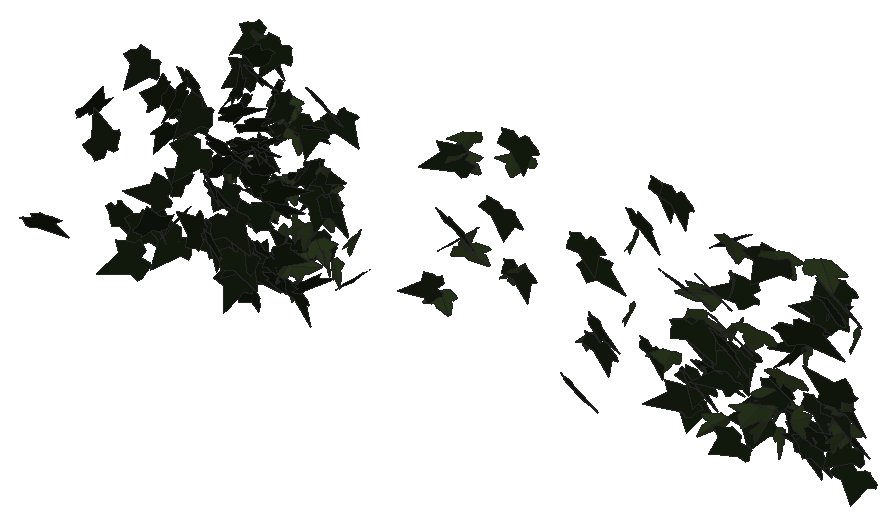
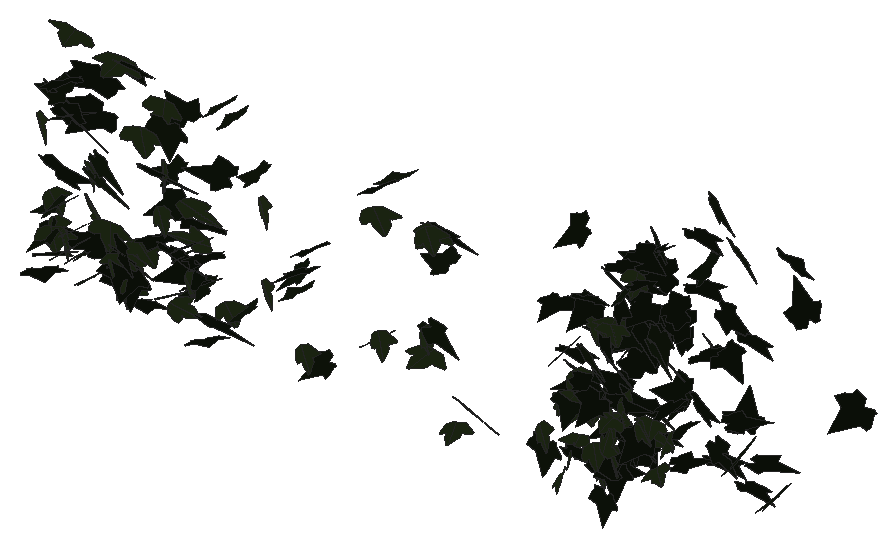
# SketchUp Ruby script. Lengths in millimetres.
U = 1.mm
M = Sketchup.active_model
def pt(a) = Geom::Point3d.new(a.map { |v| v * U })
def face(e, loops, mat)
  f = e.add_face(loops[0].map { |a| pt(a) })
  loops[1..].each { |l| e.add_face(l.map { |a| pt(a) }).erase! }
  f.material = f.back_material = mat if mat
  f
end
# faces: each face lists its corners as indices into pts; further lists are holes
def faces(e, pts, list, mat = nil) = list.each { |f| face(e, (f[0].is_a?(Array) ? f : [f]).map { |l| l.map { |i| pts[i] } }, mat) }
# xy, xz, yz: faces in a plane at the given z, y or x. An outline is a flat list of corners, or four numbers for a rectangle; further outlines are holes
def ring(l) = l.size == 4 ? [[l[0], l[1]], [l[2], l[1]], [l[2], l[3]], [l[0], l[3]]] : l.each_slice(2).to_a
def flat(e, list, mat, &to3) = list.each { |f| face(e, (f[0].is_a?(Array) ? f : [f]).map { |l| ring(l).map { |u, v| to3.(u, v) } }, mat) }
def xy(e, z, list, mat = nil) = flat(e, list, mat) { |x, y| [x, y, z] }
def xz(e, y, list, mat = nil) = flat(e, list, mat) { |x, z| [x, y, z] }
def yz(e, x, list, mat = nil) = flat(e, list, mat) { |y, z| [x, y, z] }
def lines(e, pts, list) = list.each { |a, b| e.add_line(pt(pts[a]), pt(pts[b])) }
# prism: a flat outline (further loops are holes) pulled along v
def prism(e, loops, v, mat = nil)
  f = face(e, loops, mat); d = Geom::Vector3d.new(v.map { |x| x * U })
  f.pushpull(f.normal.samedirection?(d) ? d.length : -d.length)
end
def box(e, o, s, mat = nil) = prism(e, [[o, [o[0] + s[0], o[1], o[2]], [o[0] + s[0], o[1] + s[1], o[2]], [o[0], o[1] + s[1], o[2]]]], [0, 0, s[2]], mat)
def at(x, y, z, deg = 0) = Geom::Transformation.translation(pt([x, y, z])) * Geom::Transformation.rotation(ORIGIN, Z_AXIS, deg.degrees)
def axes(o, x, y, z) = Geom::Transformation.new([*x, 0, *y, 0, *z, 0, *pt(o).to_a, 1])
def part(name) = M.definitions.add(name)
# library, detail: a bought-in or finely detailed component or shape, given as its bounding box
def library(name, o, s) = part(name).tap { |d| box(d.entities, o, s) }
def detail(e, o, s) = box(e.add_group.entities, o, s)
def put(e, d, t, mat = nil) = e.add_instance(d, t).tap { |i| i.material = mat if mat }
def group(e, t, mat = nil) = e.add_group.tap { |g| g.transformation = t; g.material = mat if mat }.entities
root = M.entities
M.materials.add("efeu1").color = [18, 25, 13]
M.materials.add("efeu2").color = [43, 57, 29]
c1 = part("ivyleaf_9")
p = [[39.1,54.8,31.7],[34.5,51.8,30.2],[-5.3,25.2,17.3],[-17.9,28.3,20.9],[-21.6,21.7,17],[-20.2,4.3,5.3],
  [-22.9,-0.3,2.5],[-17.1,-4,-0.6],[-2,-2.1,-1.2],[-0.7,-15.4,-10.1],[16.6,-22.3,-16.7],[21.1,-15.1,-12.5],
  [32.7,-10.7,-11],[46.1,-1.8,-6.6],[30.8,11.2,3.8]]
faces(c1.entities,p,[[0,1,2,3,4,5,6,7,8,9,10,11,12,13,14]],"efeu1")
c2 = part("ivyleaf_10")
p = [[0,12.8,-0.8],[-1.5,51.3,-10.9],[-4.9,51,-11.6],[-13.6,26.5,-7.3],[-13.2,15.9,-4.6],[-21.1,19.3,-7.2],
  [-29.5,16.3,-8.3],[-29.2,8.3,-6.2],[-19.7,-9.8,0.5],[-7.6,-13,4],[1,-12.2,5.8],[-0.4,51.1,-11.1],
  [-1.5,51.1,-10.9],[1,-12.4,5.9],[16.9,-12.4,3.5],[35.1,9.1,-5.1],[35,12.9,-6.1],[20.5,16.4,-4.9],
  [15.8,15,-3.8],[15.3,27.6,-7.1],[12.8,31.3,-7.8]]
faces(c2.entities,p,[[0,1,2,3,4,5,6,7,8,9,10],[11,12,0,13,14,15,16,17,18,19,20]],"efeu2")
put(root,c1,axes([93,223.6,3671.9],[1.66259,0.54862,0.30222],[0.33941,0.11819,-1.46906],[-0.68464,1.39088,0.00562]))
put(root,c1,axes([103.5,568.1,3553],[0.86385,-1.23112,-0.31612],[-0.01557,0.35496,-1.41095],[1.55061,0.68942,0.16195]))
put(root,c1,axes([180.4,600.8,4020.9],[-1.61986,-0.38705,-0.13705],[0.16378,0.02916,-1.38299],[0.4734,-1.33449,0.00953]))
put(root,c1,axes([177.8,350.7,3974.7],[0.97629,1.1061,0.65598],[-0.46966,-0.53115,1.36522],[1.49696,-0.88802,0.00051]))
put(root,c1,axes([212.5,563.8,3543.1],[-1.56561,-0.42191,0.02426],[-0.02745,-0.00923,-1.35086],[0.51485,-1.28348,0.00174]))
put(root,c1,axes([286.2,430.4,3527.5],[-1.41742,-0.52267,0.7875],[-0.87591,-0.32355,-1.27397],[0.74995,-1.36576,0.00044]))
put(root,c1,axes([299.2,523.3,3683.5],[-0.82666,-0.1305,1.15622],[-1.35744,-0.31875,-0.68804],[0.41528,-1.30168,0.05257]))
put(root,c1,axes([269.4,558.1,3580.9],[0.72765,-1.16339,-0.67837],[0.37417,-0.60509,1.30737],[-1.59984,-0.67066,-0.00278]))
put(root,c1,axes([342,503.3,4001.5],[-0.41991,0.20999,-1.38623],[-1.63505,-0.46852,0.26179],[-0.50239,1.34929,0.30664]))
put(root,c1,axes([321,522.1,3900.5],[-0.02006,1.00641,-0.92606],[0.06724,-0.92488,-1.00611],[-1.66716,-0.04941,-0.02943]))
put(root,c1,axes([330,548.8,3617.5],[-0.7977,0.991,-0.59397],[0.30979,-0.54255,-1.18473],[-1.37509,-0.69712,0.07767]))
put(root,c1,axes([341.5,530.6,3565.5],[-1.64628,-0.66672,0.05597],[-0.06226,-0.02307,-1.50513],[0.81388,-1.35037,-0.00192]))
put(root,c1,axes([324.7,436.7,3628.8],[1.05978,0.58087,1.00057],[-0.9984,-0.57596,1.04485],[0.99775,-1.19332,-0.01725]))
put(root,c1,axes([367.3,187,4002],[-1.75311,0.25356,-0.39672],[-0.49078,0.00084,1.45765],[0.29846,1.49073,0.06665]))
put(root,c1,axes([344.5,596.9,3909.2],[-0.8173,-1.09414,0.35514],[-0.1806,-0.32555,-1.28224],[1.39173,-0.68478,0.04216]))
put(root,c2,axes([359.2,722.5,3691],[-0.07252,0.88199,-0.84663],[-0.03391,-0.84839,-0.88187],[-1.49116,-0.02361,0.06123]))
put(root,c1,axes([413.5,358.1,4101.2],[-0.92706,1.06786,0.64427],[-0.41717,0.54714,-1.31017],[-1.46323,-0.83256,-0.03466]))
put(root,c1,axes([418.2,603.6,3551.2],[-0.82674,-0.26939,1.09771],[-1.16682,-0.54541,-0.72428],[0.73486,-1.16907,0.08495]))
put(root,c1,axes([425.2,667.2,3975],[-0.28819,1.2174,0.3214],[-0.09797,0.31177,-1.23996],[-1.53299,-0.24879,0.01882]))
put(root,c1,axes([444.7,418.8,3814.2],[-0.58367,0.80905,1.0484],[-0.68559,0.88534,-0.93966],[-1.46293,-0.7377,0.02208]))
put(root,c2,axes([446.3,734.4,3715.3],[-0.43296,0.28503,1.11686],[-1.332,0.29158,-0.42134],[-0.45091,-1.13504,0.17223]))
put(root,c2,axes([410.3,721.3,3733.4],[1.37324,0.39307,0.26807],[0.30309,0.10164,-1.19218],[-0.49504,1.15261,0.01371]))
put(root,c1,axes([445.4,676.6,3935.4],[-0.98878,0.97289,0.13476],[-0.08816,0.11517,-1.26612],[-1.19501,-0.81349,-0.01809]))
put(root,c1,axes([404.2,485.2,4102.8],[1.07559,-1.14499,0.24024],[0.18253,-0.188,-1.44508],[1.41558,0.89423,0.00379]))
put(root,c1,axes([468.7,458.6,3657.4],[-1.00509,0.13634,-1.1871],[-1.45682,-0.04146,0.82395],[0.05306,1.44437,0.1357]))
put(root,c1,axes([464,729.3,4138.8],[-1.26349,-0.55013,0.4761],[-0.46885,-0.28961,-1.1706],[0.75366,-1.10243,0.06994]))
put(root,c2,axes([451.2,649.4,3541.6],[0.59396,1.1013,-0.37433],[-0.16721,-0.34865,-1.20402],[-1.40919,0.50556,-0.01492]))
put(root,c1,axes([445.3,589,3720.8],[0.35921,-0.93222,-0.91034],[-0.04156,0.92747,-0.96078],[1.58909,0.23498,0.18066]))
put(root,c2,axes([489.2,642.8,3639.4],[0.56682,0.67833,-0.96279],[-1.11146,-0.44894,-0.75593],[-0.91062,0.97019,0.32336]))
put(root,c1,axes([464.5,553.9,3618],[-0.38114,-1.44345,0.12125],[0.05723,-0.13405,-1.47502],[1.76629,-0.30714,0.07396]))
put(root,c2,axes([479.3,707.7,4147],[-1.52341,0.20497,-0.02115],[0.01482,-0.05646,-1.26426],[-0.25096,-1.2476,0.05374]))
put(root,c1,axes([444.2,546.8,3733.7],[1.24955,-0.74101,0.78859],[0.79403,-0.44562,-1.26405],[1.0547,1.21339,0.01737]))
put(root,c1,axes([475.9,676.9,3644.9],[1.40341,0.58383,0.06138],[0.05357,0.04908,-1.28979],[-0.71419,1.15093,0.02386]))
put(root,c1,axes([529.3,563.5,3852.1],[-1.41301,0.86921,0.23179],[-0.27701,0.08317,-1.44646],[-1.06196,-1.17824,0.06889]))
put(root,c1,axes([490.6,721.7,4117.2],[0.92204,-0.99232,-0.24267],[-0.22677,0.16325,-1.24643],[1.2255,0.77681,-0.04806]))
put(root,c2,axes([517.7,788.7,3645.6],[-1.29428,0.52073,-0.11674],[-0.12291,0.05968,1.18176],[0.63936,1.06562,-0.00914]))
put(root,c1,axes([526.9,381.8,3963.6],[-1.45086,-0.86005,0.10812],[-0.1181,-0.05064,-1.46755],[1.0509,-1.19306,-0.01565]))
put(root,c1,axes([544.9,729.8,3876.4],[-0.90397,0.82574,0.5679],[-0.46842,0.41848,-1.10943],[-1.12937,-0.83451,0.00559]))
put(root,c1,axes([534.5,575.4,3909.6],[0.62605,1.03145,-0.63629],[-0.46787,-0.51727,-1.1478],[-1.40256,0.63295,0.09887]))
put(root,c1,axes([535.2,766.3,3485.1],[0.07755,1.15918,0.3041],[0.00165,0.30446,-1.16083],[-1.46205,0.06183,0.01482]))
put(root,c1,axes([538.2,304,4178.9],[-1.39021,0.73613,-0.62099],[0.64798,-0.32215,-1.35651],[-0.98012,-1.25712,-0.01601]))
put(root,c1,axes([539.8,623.9,4162],[-0.21576,0.48602,-1.27275],[0.15229,-1.27225,-0.50317],[-1.65512,-0.18041,0.11962]))
put(root,c1,axes([516.9,439.2,3662.9],[1.44529,-0.50835,-0.63513],[-0.66556,0.33587,-1.28639],[0.73624,1.30154,0.0839]))
put(root,c1,axes([515.2,450.7,3813.2],[-0.15247,-0.22861,1.35165],[0.46584,-1.30935,-0.18615],[1.60625,0.35803,0.18229]))
put(root,c1,axes([515.7,443.4,3871.4],[0.53305,0.10982,1.41408],[1.28934,0.96162,-0.40122],[-1.15404,1.12509,0.2049]))
put(root,c1,axes([502.3,476.5,3933.4],[1.42172,-0.32839,0.64756],[0.75704,-0.18536,-1.2107],[0.45992,1.32023,-0.00891]))
put(root,c1,axes([548.7,362.9,4108.3],[-1.687,-0.46875,-0.09816],[0.11756,0.02149,-1.46004],[0.57233,-1.3861,0.01056]))
put(root,c1,axes([566.8,578.6,3551.8],[-0.24974,0.90108,1.06087],[-0.86299,0.85614,-0.86368],[-1.46248,-0.65907,0.32848]))
put(root,c1,axes([549,565.5,4128.5],[-0.80598,-0.68803,0.88155],[-0.41967,-0.84921,-0.92058],[1.29813,-0.70172,0.24973]))
put(root,c1,axes([578.8,672.8,3714.4],[-0.99396,0.12778,0.98929],[-1.20044,0.10681,-0.82414],[-0.19984,-1.27713,0.03006]))
put(root,c1,axes([555.2,690.1,4153.2],[-1.12697,-0.92692,0.09963],[-0.08098,-0.0745,-1.30861],[1.13447,-0.92611,0.00556]))
put(root,c1,axes([534.9,603.2,3803.2],[1.4637,0.61452,0.39653],[-0.4653,-0.12432,1.34661],[0.76131,-1.25746,0.06065]))
put(root,c2,axes([530,745.2,3709.9],[1.20405,0.29131,0.68503],[0.8041,0.1868,-1.029],[-0.42213,1.18676,-0.00618]))
put(root,c2,axes([546.2,720.2,3974.2],[1.43009,0.4523,-0.07607],[-0.07405,-0.05395,-1.25611],[-0.55463,1.17343,-0.02843]))
put(root,c1,axes([524.4,558.7,3897.1],[1.35354,0.20211,0.77368],[0.9036,0.23905,-1.12455],[-0.36775,1.33129,0.08447]))
put(root,c2,axes([552.3,723.3,3680.9],[-0.35582,0.09054,-1.21967],[-0.09008,-1.25289,-0.07535],[-1.48938,0.05415,0.29594]))
put(root,c1,axes([563.7,688.9,3525],[0.61115,1.04363,-0.38049],[-0.27439,-0.31346,-1.15588],[-1.32715,0.5454,0.06376]))
put(root,c1,axes([552.3,689.5,4032.1],[-0.48176,0.23985,-1.23143],[1.10937,-0.83472,-0.45418],[-1.05451,-0.98773,0.08479]))
put(root,c2,axes([560.1,708.6,3578.4],[0.96038,-0.88646,-0.20753],[-0.14207,0.17406,-1.1852],[1.1016,0.79527,0.02807]))
put(root,c2,axes([562,664.1,3682.8],[1.1327,-0.7396,-0.28525],[-0.27826,0.17149,-1.18699],[0.9262,0.95601,-0.00776]))
put(root,c1,axes([569,724.8,3897.8],[0.50175,-0.28071,1.15398],[-0.41451,1.14236,0.39898],[-1.38835,-0.44252,0.29793]))
put(root,c2,axes([551.5,673.1,3725.7],[-0.2369,-0.48725,1.13069],[0.59128,-1.0825,-0.38325],[1.38081,0.37994,0.3581]))
put(root,c1,axes([543.2,588.6,3661],[-0.72927,0.14735,1.18784],[1.40937,-0.27647,0.61564],[0.38219,1.30071,-0.00371]))
put(root,c1,axes([551.4,556.1,3975.1],[1.1143,0.85435,0.43133],[0.35299,0.32184,-1.25016],[-1.11297,0.95744,0.03535]))
put(root,c1,axes([541,483.3,4034.7],[0.94564,0.32705,1.07998],[1.05053,0.67535,-0.82253],[-0.88973,1.14501,0.17667]))
put(root,c1,axes([575,482.7,4106.1],[0.337,0.21539,1.30342],[-0.20965,1.32615,-0.18272],[-1.59805,-0.12856,0.29884]))
put(root,c1,axes([553.9,606.8,3894.7],[0.95347,-0.78906,-0.71759],[-0.52146,0.58335,-1.10696],[1.19215,0.88625,0.08972]))
put(root,c1,axes([536.5,585.2,4117.1],[0.82005,-0.66735,0.87858],[0.93174,-0.46103,-0.93449],[0.97141,1.00557,0.15464]))
put(root,c1,axes([587.8,717.1,3522.4],[0.50144,-0.01919,1.19464],[-1.43925,0.19356,0.40899],[-0.23084,-1.24845,0.04505]))
put(root,c1,axes([575.3,667.1,3498.7],[-0.05426,-0.31006,-1.22847],[0.37321,-1.19549,0.29066],[-1.5,-0.28623,0.11675]))
put(root,c1,axes([567.6,592.6,3899.6],[0.81921,0.8277,0.75502],[0.29681,0.75151,-1.04022],[-1.33418,0.67541,0.23218]))
put(root,c1,axes([574.1,492.1,3546.6],[-1.46393,-0.5015,-0.53202],[0.66592,0.06578,-1.29311],[0.59343,-1.31095,0.13864]))
put(root,c1,axes([558.6,592.1,3531.5],[-0.04939,-0.64148,-1.07577],[0.22625,1.0614,-0.63989],[1.51122,-0.17987,0.06064]))
put(root,c2,axes([561.1,700.6,3979.3],[0.88966,0.93638,0.44496],[0.3701,0.32747,-1.1863],[-1.20944,0.789,-0.0357]))
put(root,c1,axes([586.8,582.7,3589.4],[0.92592,0.12806,-1.02845],[-1.24351,-0.1385,-0.76942],[-0.22886,1.27064,0.01978]))
put(root,c1,axes([599.1,506.1,3516.7],[0.74294,0.08753,-1.29393],[-1.56293,-0.18182,-0.61522],[-0.24618,1.41846,0.00099]))
put(root,c1,axes([578.2,743.1,3753.9],[1.0389,0.8684,0.2679],[0.20997,0.20639,-1.21607],[-1.08866,0.86852,0.02111]))
put(root,c1,axes([612.4,495.4,3624.8],[-1.72149,0.21487,-0.05452],[0.0658,-0.00797,-1.42733],[-0.26233,-1.41209,-0.00024]))
put(root,c2,axes([597.3,737.6,3596],[-0.72009,-1.06919,0.12767],[0.03242,-0.16001,-1.21719],[1.31328,-0.5823,0.10005]))
put(root,c1,axes([577.9,482.3,3620.8],[0.13069,-1.33487,-0.47382],[0.5898,0.4811,-1.24607],[1.62432,-0.06729,0.49058]))
put(root,c1,axes([582.4,537.4,3804.6],[-0.39568,0.02926,1.27197],[1.07298,-0.94337,0.24596],[1.12164,0.91277,0.21343]))
put(root,c2,axes([631.4,639.1,3540.5],[0.23125,0.7399,-0.97327],[-0.37167,-0.92525,-0.76273],[-1.44451,0.35651,0.04044]))
put(root,c1,axes([601.6,597.7,3501.6],[0.87243,0.43704,-0.94075],[1.00948,0.44877,0.83746],[0.76322,-1.09316,-0.03231]))
put(root,c1,axes([602.4,610.2,3720.6],[0.46402,-0.47525,1.13365],[1.28534,-0.48532,-0.55693],[0.7726,1.09283,0.24567]))
put(root,c1,axes([655.7,601.9,4051.5],[-1.51646,0.36607,-0.1268],[0.14379,-0.04862,-1.29571],[-0.45023,-1.2485,0.01328]))
put(root,c1,axes([622.9,383,3787.9],[0.05754,-1.06233,-1.02471],[0.14925,1.02452,-1.0565],[1.79452,-0.05114,0.12072]))
put(root,c2,axes([633.3,671.5,3930.5],[1.50558,0.00638,0.19622],[0.23582,0.17878,-1.22154],[-0.04185,1.23673,0.17557]))
put(root,c2,axes([648.2,650.3,3484.7],[0.17183,-1.20988,0.01144],[0.00804,-0.01075,-1.21804],[1.4761,0.1409,0.00531]))
put(root,c1,axes([633,574.2,3594.4],[0.22923,0.1676,-1.27506],[-0.1174,1.28682,0.15497],[1.56456,0.072,0.19844]))
put(root,c1,axes([624.9,723.5,3785.6],[0.52282,-0.09339,-1.18657],[0.46167,1.20639,0.04172],[1.37675,-0.36908,0.43661]))
put(root,c2,axes([652.7,633.3,3664],[0.3701,-0.50496,-1.11947],[0.02532,1.15506,-0.51539],[1.49805,0.10523,0.28528]))
put(root,c1,axes([675,743.7,3570.7],[-1.4127,-0.21931,0.1775],[-0.21906,-0.00554,-1.17821],[0.2655,-1.17146,-0.02766]))
put(root,c2,axes([663.9,728.6,3792],[-0.51812,-1.13415,0.37068],[-0.01718,-0.38867,-1.20532],[1.45559,-0.40829,0.11772]))
put(root,c1,axes([671.8,746.6,3725.3],[0.31073,1.17838,0.31632],[-0.00174,0.32343,-1.2037],[-1.48851,0.24561,0.06744]))
put(root,c2,axes([653,649.4,3536.3],[0.02251,-0.3794,-1.17494],[0.96542,0.90563,-0.28001],[1.15625,-0.74877,0.25667]))
put(root,c1,axes([694.6,661.8,3830.9],[-1.14636,0.84628,-0.01275],[0.0118,-0.00831,-1.26456],[-1.03251,-0.93969,-0.0003]))
put(root,c2,axes([667.5,740.8,3730],[0.82239,0.78266,0.71109],[0.39012,0.65293,-1.02178],[-1.22969,0.73057,0.1514]))
put(root,c2,axes([687.2,662.6,3658.7],[-0.10557,-1.15633,0.42915],[0.09363,-0.43442,-1.15505],[1.50183,-0.0542,0.10218]))
put(root,c2,axes([678.2,703.4,3584.3],[0.736,0.97589,0.42223],[0.12105,0.43168,-1.13948],[-1.29159,0.59656,0.13382]))
put(root,c2,axes([684.7,765.8,3497.2],[-0.34564,1.18421,-0.03155],[0.01013,-0.03045,-1.21762],[-1.44521,-0.28343,-0.00099]))
put(root,c1,axes([677.5,642.7,3965.5],[1.32659,0.67683,0.16824],[0.14888,0.12217,-1.28022],[-0.83774,1.0935,0.0389]))
put(root,c1,axes([663.3,514.4,3828.8],[0.62229,0.70814,-1.0652],[0.55007,0.97362,0.86317],[1.46034,-0.6685,0.12878]))
put(root,c2,axes([693,712.6,3685.3],[-1.43291,-0.34539,-0.19391],[0.21135,0.09777,-1.22345],[0.43458,-1.1864,-0.04437]))
put(root,c2,axes([695.2,710.2,3552.9],[-0.77459,1.00602,0.25695],[-0.22972,0.18462,-1.18814],[-1.24574,-0.65958,0.05933]))
put(root,c1,axes([708.2,688.5,3787.2],[-1.48386,0.04784,-0.31719],[0.37553,-0.17592,-1.20687],[-0.11012,-1.24459,0.1584]))
put(root,c1,axes([698.3,652.4,3985.3],[-1.08093,-0.83086,-0.43582],[0.46469,0.22929,-1.21146],[1.04607,-0.96041,0.08781]))
put(root,c1,axes([736.5,712,3992.9],[-0.15365,-0.77016,-1.0234],[0.25177,1.0027,-0.77997],[1.54218,-0.24043,0.02537]))
put(root,c2,axes([755.5,762.3,3610.7],[0.08231,-1.22382,-0.02856],[-0.04984,0.02633,-1.22505],[1.49264,0.06836,-0.03933]))
put(root,c1,axes([756.8,629.1,3794.8],[-1.22762,-0.86669,-0.42684],[0.61971,0.04963,-1.29823],[1.00258,-1.09191,0.2798]))
put(root,c1,axes([795.1,692.9,3522.6],[0.23399,1.24661,0.32281],[-0.13314,0.34093,-1.25175],[-1.56538,0.15734,0.15472]))
put(root,c1,axes([768.4,567.7,4137.2],[1.63088,-0.52591,-0.02799],[-0.03138,0.01108,-1.43652],[0.64176,1.33704,0.00089]))
put(root,c1,axes([770.6,488.7,3575.7],[0.70243,-1.259,0.49878],[0.28059,-0.4432,-1.38422],[1.62813,0.61956,0.02336]))
put(root,c1,axes([777.5,622.2,3790.4],[0.73364,-1.17618,-0.37828],[-0.09319,0.3845,-1.31698],[1.50444,0.59738,0.10289]))
put(root,c1,axes([796.3,477.1,3596.9],[0.92993,0.71598,1.0492],[0.70039,0.89732,-1.02941],[-1.38236,0.93629,0.18424]))
put(root,c1,axes([1054,732.6,3573.1],[-1.72421,0.6776,0.16824],[-0.35931,0.02758,-1.12774],[-1.27925,-0.92103,0.09]))
put(root,c2,axes([1036.6,778.3,3526.4],[-1.00157,-0.98427,-0.1825],[0.74258,-0.0118,-1.06145],[1.75453,-0.55688,0.34506]))
put(root,c1,axes([1156.9,733.3,3770.4],[-0.91441,0.93746,-0.52932],[0.20411,-0.53508,-1.045],[-2.03874,-0.47404,0.13279]))
put(root,c2,axes([1152.5,752.3,4064.6],[-0.9738,-1.07479,0.19416],[0.03838,-0.22367,-1.18501],[2.0783,-0.49947,0.11286]))
put(root,c2,axes([1137.8,766.4,3709.7],[-1.55832,-0.54362,-0.64582],[1.08957,0.3036,-0.98138],[1.1807,-0.99766,0.05326]))
put(root,c2,axes([1154.8,760.1,3761.3],[0.02819,-1.17512,0.06251],[0.16189,-0.06129,-1.17219],[2.23379,0.01927,0.08416]))
put(root,c1,axes([1189,679.6,4038],[-2.22138,0.14608,0.27419],[-0.5181,0.03276,-1.17629],[-0.28492,-1.19851,0.00126]))
put(root,c2,axes([1179.9,687,4034.4],[-1.36512,-0.73165,-0.63379],[0.95678,0.39253,-1.02209],[1.57433,-0.87298,0.0716]))
put(root,c1,axes([1202.5,604.9,3889.6],[0.8226,-0.99904,0.53344],[0.56214,-0.45177,-1.08541],[2.08085,0.51698,0.08234]))
put(root,c2,axes([1302.6,767.4,3700.5],[-0.50102,-1.11937,-0.16844],[0.02732,0.16962,-1.14964],[2.15419,-0.26249,-0.0246]))
put(root,c1,axes([1302.5,774.7,3701.7],[0.02554,-1.16177,0.09011],[0.01844,-0.09,-1.16182],[2.21765,0.01413,0.00862]))
put(root,c2,axes([1335,745.4,4060.1],[-1.45208,-0.8833,0.30452],[-0.22495,-0.29874,-1.16269],[1.7639,-0.76525,0.10241]))
put(root,c1,axes([1341.8,726.6,4130.8],[-0.28328,-1.21491,0.03913],[-0.01788,-0.03827,-1.22399],[2.31335,-0.14907,-0.00467]))
put(root,c1,axes([1442.2,534.9,4032.4],[-0.59016,-1.11283,0.47862],[0.26485,-0.5235,-1.12703],[2.29025,-0.22622,0.25366]))
put(root,c2,axes([1545.9,787,3581.7],[-0.39819,-1.13014,-0.01788],[-0.00862,0.01902,-1.14932],[2.15114,-0.20912,-0.00792]))
put(root,c1,axes([1548.8,753.6,3880],[-0.13521,-1.18727,-0.06644],[-0.01247,0.06695,-1.18934],[2.26311,-0.07057,-0.01052]))
put(root,c1,axes([1558.9,668,3491.2],[1.86851,-0.54869,-0.35898],[-0.51448,0.25016,-1.12167],[1.13692,1.01497,0.0824]))
put(root,c1,axes([1564.3,763.1,3814],[0.66449,-0.86934,-0.72445],[0.09666,0.76942,-0.89883],[2.15155,0.23392,0.26412]))
put(root,c1,axes([1663.3,641.3,3723.8],[1.52637,-0.75694,-0.50991],[-0.63791,0.3871,-1.10181],[1.61562,0.86797,0.04671]))
put(root,c2,axes([1692.5,767.5,3717.5],[0.44393,-1.14394,-0.09887],[-0.03066,0.09762,-1.16747],[2.18504,0.23378,0.0037]))
put(root,c1,axes([1675.7,654.4,3655.5],[-0.03202,-1.13373,0.40994],[0.21213,-0.40968,-1.12845],[2.2846,0.02215,0.11053]))
put(root,c2,axes([1717.8,750.3,3954],[0.37707,-1.16682,-0.20693],[-0.00176,0.20965,-1.18304],[2.25534,0.19525,0.03367]))
put(root,c1,axes([1740.8,735.9,4030.1],[0.83336,-1.1213,0.19248],[0.07975,-0.19021,-1.20339],[2.1638,0.43887,-0.02978]))
put(root,c1,axes([1757.6,776.6,3617.2],[0.22794,-1.02798,0.52313],[0.1653,-0.51641,-1.03466],[2.18898,0.14604,0.02366]))
put(root,c2,axes([1813.4,777.1,3616.3],[-1.08962,-0.9368,0.37642],[0.01316,-0.43636,-1.07545],[1.92142,-0.52826,0.22083]))
put(root,c1,axes([1841.4,721.3,4155.7],[0.11982,-1.12647,0.5068],[0.0008,-0.50744,-1.12795],[2.35089,0.05759,-0.02545]))
put(root,c1,axes([1913.3,741.4,3530.7],[-2.16159,0.158,0.39255],[-0.74661,0.02835,-1.14644],[-0.30191,-1.20136,0.02457]))
put(root,c1,axes([1888,786.3,3497],[-0.86555,-1.05416,0.10034],[-0.03197,-0.102,-1.14781],[2.01509,-0.45442,0.02489]))
put(root,c1,axes([1899.2,766.8,3740.6],[-0.25376,-1.08675,-0.43796],[0.13262,0.43265,-1.09479],[2.22599,-0.14967,0.0153]))
put(root,c1,axes([1897.1,703.9,4166.3],[0.10603,-1.20049,0.29909],[0.0311,-0.29865,-1.20178],[2.3544,0.05801,0.0024]))
put(root,c2,axes([1962.8,754.2,3865],[1.15212,0.03725,-1.03146],[-1.94164,0.2029,-0.59142],[0.29784,1.17864,0.13441]))
put(root,c1,axes([1922.1,728.7,3619],[1.2792,-1.01656,-0.05675],[-0.06354,0.04595,-1.21867],[1.93669,0.67296,-0.0025]))
put(root,c1,axes([1906.7,666,3933.8],[1.52804,-0.77938,0.55092],[0.98047,-0.25216,-1.10751],[1.52914,0.9405,0.1596]))
put(root,c2,axes([1912.8,761.1,3770],[0.26714,0.03807,1.1742],[2.18285,0.25168,-0.14526],[-0.48426,1.15547,-0.00704]))
put(root,c2,axes([1954.6,767.8,3645.7],[0.55041,-1.04183,0.45253],[0.41774,-0.40691,-1.07707],[2.12103,0.3505,0.0947]))
put(root,c1,axes([1934.8,760.2,3763.9],[0.49778,-1.05452,-0.46703],[0.16451,0.49547,-1.07032],[2.18882,0.20258,0.18666]))
put(root,c1,axes([1957.4,730.4,3615.3],[-0.77177,-1.05086,0.29037],[-0.09324,-0.29193,-1.12492],[2.07286,-0.40439,0.05751]))
put(root,c1,axes([1960.3,760.1,3724.6],[0.24736,-1.16541,0.11002],[-0.02933,-0.11239,-1.17231],[2.22768,0.12793,-0.02765]))
put(root,c1,axes([1957.4,702.2,3788.5],[-0.69072,-0.93566,-0.71448],[1.39235,0.40652,-0.90398],[1.75541,-0.69061,0.43588]))
put(root,c1,axes([1961.9,734.6,3654.8],[2.21957,-0.32753,0.1954],[0.3499,-0.06798,-1.21125],[0.63595,1.18053,-0.01554]))
put(root,c1,axes([2013.6,765.9,3720],[-2.17508,-0.09267,-0.27996],[0.53103,0.02292,-1.14661],[0.18169,-1.17642,-0.00028]))
put(root,c2,axes([2032.6,719.5,3518.6],[-0.38126,-0.71324,0.96606],[-0.31029,-0.95419,-0.73828],[2.26425,-0.25086,0.0615]))
put(root,c1,axes([2051.8,734.1,4068.8],[0.43151,1.19784,0.11087],[0.00888,0.11195,-1.219],[-2.28945,0.2262,0.01617]))
put(root,c1,axes([2088.3,702.7,3671.1],[-2.0001,0.44694,0.30048],[-0.54751,0.09112,-1.14167],[-0.86649,-1.08922,0.02779]))
put(root,c2,axes([2061.9,753.7,3806.8],[-0.18974,-1.18923,-0.09221],[0.02744,0.09133,-1.19339],[2.26998,-0.10051,0.00672]))
put(root,c2,axes([2058.2,739.9,3943.9],[0.74621,-1.0027,-0.54799],[0.07542,0.59093,-1.05292],[2.17342,0.32375,0.22468]))
put(root,c1,axes([2032.6,707.7,3828.5],[2.0473,-0.63641,-0.05333],[-0.07859,0.03493,-1.24984],[1.21292,1.07647,0.00903]))
put(root,c1,axes([2111.4,747.4,3921],[-1.92655,0.41714,0.51111],[-1.07164,-0.0585,-1.06745],[-0.65428,-1.13247,0.24341]))
put(root,c1,axes([2069.2,754.1,3731.9],[-0.50141,-1.07919,-0.40375],[0.20463,0.38934,-1.11082],[2.18338,-0.28432,0.01139]))
put(root,c1,axes([2070.2,724.6,3722.7],[-0.13195,-1.12895,-0.51525],[0.05919,0.51431,-1.13108],[2.36107,-0.07599,-0.00044]))
put(root,c2,axes([2103.7,691.6,4094.7],[-2.24214,0.31352,0.14915],[-0.28012,0.02687,-1.21904],[-0.59845,-1.18719,0.0118]))
put(root,c1,axes([2122.2,687.3,3497.4],[-1.417,-0.56698,0.78751],[-0.56629,-0.8114,-0.86549],[1.75787,-0.71842,0.35599]))
put(root,c1,axes([2123.5,772.7,3528.7],[-1.64656,-0.74424,-0.24341],[0.52698,0.04853,-1.13253],[1.394,-0.89743,0.14062]))
put(root,c2,axes([2145.8,771.7,3564.4],[-0.64622,-1.03795,-0.42553],[0.23723,0.40694,-1.09205],[2.12178,-0.36162,-0.0075]))
put(root,c1,axes([2111.1,582.5,4005.6],[0.10616,-0.72625,1.04556],[0.90806,-0.95836,-0.69113],[2.24626,0.42174,0.22998]))
put(root,c1,axes([2162.1,770,3586.6],[0.94022,0.99682,-0.37978],[-0.24745,-0.35914,-1.11178],[-2.01504,0.50922,-0.04068]))
put(root,c1,axes([2121.9,611.8,3846.1],[1.06108,-1.04352,0.42032],[0.31379,-0.38825,-1.18259],[2.11797,0.58031,-0.03537]))
put(root,c1,axes([2164.5,765.9,3599.9],[1.30932,0.94268,-0.15589],[-0.20947,-0.11263,-1.16681],[-1.80638,0.69635,0.02231]))
put(root,c2,axes([2183.7,765.2,3630.4],[1.92212,0.49951,-0.35423],[-0.81189,0.08373,-1.09817],[-0.83613,1.06698,0.25201]))
put(root,c1,axes([2209.9,760.9,3644.6],[-2.11338,0.40907,0.08257],[-0.17287,-0.00782,-1.18275],[-0.7752,-1.11347,0.03864]))
put(root,c2,axes([2194.5,673.3,3628.1],[-1.55643,-0.78869,0.50414],[-0.43047,-0.48311,-1.12269],[1.72871,-0.83039,0.17434]))
put(root,c1,axes([2214.4,761.3,3673.8],[0.56408,0.01036,-1.15019],[-2.18899,0.01616,-0.29623],[0.02487,1.18766,0.01407]))
put(root,c2,axes([2206.6,688.4,3581.6],[0.00206,-1.16186,0.1635],[0.00647,-0.1635,-1.16186],[2.23303,0.00155,0.00322]))
put(root,c2,axes([2207.9,766,3607.3],[0.11125,-1.17459,0.00428],[-0.0348,-0.00519,-1.1759],[2.23522,0.05838,-0.01852]))
put(root,c2,axes([2233.9,756.8,3704],[-2.24441,-0.06347,0.16864],[-0.32059,-0.00821,-1.18099],[0.12179,-1.19125,-0.00085]))
put(root,c2,axes([2253.8,600.1,3915.9],[-2.23564,-0.14325,0.28175],[-0.51412,-0.10795,-1.18116],[0.31231,-1.20316,0.07243]))
put(root,c2,axes([2242.4,719.9,3548.9],[1.19173,-0.91261,0.47756],[0.6677,-0.3365,-1.10304],[1.8431,0.71199,0.09081]))
put(root,c1,axes([2303.1,742.2,3838.4],[-1.54466,0.89778,0.03497],[-0.27667,-0.08472,-1.19902],[-1.68743,-0.80793,0.16458]))
put(root,c1,axes([2284.7,641.8,4136],[-2.24946,-0.31854,-0.22534],[0.44931,-0.01147,-1.22203],[0.59125,-1.20317,0.07131]))
put(root,c1,axes([2265.7,773.3,3555.3],[0.5195,-1.11304,-0.23533],[-0.00042,0.24196,-1.14464],[2.16517,0.26711,0.05624]))
put(root,c2,axes([2289.3,644.6,4143.6],[-2.08831,-0.35053,-0.47335],[0.96607,-0.05507,-1.13588],[0.56865,-1.19374,0.1914]))
put(root,c1,axes([2329.6,690.4,3850.4],[-1.31187,0.92152,-0.45373],[0.49187,-0.37326,-1.15069],[-1.89201,-0.73599,0.01546]))
put(root,c2,axes([2305.3,740.7,3839.2],[-1.12986,0.84866,-0.62841],[0.06157,-0.70595,-0.98394],[-2.00882,-0.49896,0.32329]))
put(root,c1,axes([2360.5,700.5,3573.5],[1.25746,0.00933,1.06659],[-1.92065,0.41171,0.62154],[-0.6573,-1.18518,0.22431]))
put(root,c1,axes([2383.3,727.2,3975.4],[-1.43624,0.87748,0.41902],[-0.55794,0.30042,-1.15709],[-1.76456,-0.80921,0.02481]))
put(root,c1,axes([2342.8,755.4,3663.9],[-0.07212,-1.17991,0.08695],[-0.00171,-0.08696,-1.18052],[2.25169,-0.03786,0.00189]))
put(root,c2,axes([2336.4,668.2,3649.4],[0.88163,-0.79609,-0.84419],[0.95616,-0.68176,0.91859],[-1.99066,-0.68004,0.06734]))
put(root,c1,axes([2344.5,696.8,3570.8],[0.42912,-1.15207,-0.01706],[-0.03095,0.0142,-1.17386],[2.19265,0.22567,-0.01323]))
put(root,c1,axes([2352.8,698.1,3572.8],[0.7552,-1.01679,-0.4335],[-0.25336,0.41328,-1.0912],[2.08838,0.41783,0.02438]))
put(root,c1,axes([2352.9,743.9,3605.1],[0.83255,-0.94854,-0.54517],[-0.19784,0.54844,-1.03764],[2.07277,0.43334,0.11993]))
put(root,c2,axes([2383,761.2,3623.9],[0.61987,-1.12558,-0.10672],[0.14596,0.1328,-1.16657],[2.14686,0.31596,0.11012]))
put(root,c1,axes([2362.7,631.6,3959.5],[2.22961,0.49443,0.1404],[0.25846,0.03927,-1.27146],[-0.94345,1.17923,-0.01653]))
put(root,c1,axes([2401.1,728.3,3975.2],[-1.10297,-1.05101,0.26688],[0.02905,-0.31049,-1.18957],[2.06356,-0.55739,0.1594]))
put(root,c1,axes([2388.7,729.5,3976.1],[-0.37909,0.21932,1.19503],[1.16635,-1.02751,0.29073],[1.99666,0.64186,0.05706]))
put(root,c2,axes([2432.4,754.1,3621.7],[-1.60532,-0.7947,0.20262],[0.03913,-0.31106,-1.13442],[1.56038,-0.80979,0.23691]))
put(root,c1,axes([2438.1,763.9,3558],[-1.51464,-0.74014,0.43182],[-0.27083,-0.46699,-1.06269],[1.6082,-0.77572,0.22773]))
put(root,c1,axes([2476.6,675.6,3757.5],[-0.26737,0.33413,1.23215],[-1.59898,0.90913,-0.34233],[-1.82942,-0.84345,0.11913]))
put(root,c1,axes([2416.4,728.8,3701.5],[0.29036,-1.17498,-0.12702],[0.00517,0.12842,-1.18469],[2.24925,0.15139,0.01912]))
put(root,c1,axes([2424.4,719.8,4068.2],[-0.27277,-1.18606,-0.3426],[0.09313,0.33917,-1.19466],[2.34774,-0.15126,0.00758]))
put(root,c2,axes([2450.9,713.4,3624],[-0.18388,-1.17079,0.08957],[-0.01816,-0.08909,-1.17477],[2.23468,-0.09706,-0.00218]))
put(root,c2,axes([2451.2,725.3,3712.7],[-0.56897,-1.08825,0.36496],[0.06357,-0.38523,-1.12132],[2.1836,-0.27235,0.12774]))
put(root,c1,axes([2420.8,749.4,3703.1],[0.99668,-1.06756,-0.00366],[0.00606,0.00564,-1.18908],[2.03178,0.52367,0.00534]))
put(root,c1,axes([2415.8,722.5,4037.9],[1.04972,-0.95488,0.56496],[0.53703,-0.48944,-1.10273],[2.04216,0.61954,-0.00041]))
put(root,c1,axes([2435.3,747.1,3624.9],[1.70411,-0.65015,-0.55073],[-0.81797,0.3452,-1.10627],[1.40021,0.99291,0.024]))
put(root,c1,axes([2424.2,554.6,4012.2],[-0.14833,-0.1337,-1.35641],[1.64354,1.04628,-0.15275],[2.00692,-0.86672,0.02484]))
put(root,c1,axes([2467.1,757.8,3495.1],[-1.03375,-1.01854,-0.09949],[0.02852,0.1047,-1.15376],[1.9475,-0.54218,-0.03591]))
put(root,c2,axes([2447.2,636.2,4172.5],[2.22929,0.08212,0.48523],[0.9166,0.06634,-1.17383],[-0.19262,1.26613,0.03003]))
put(root,c2,axes([2491.2,728,3930.8],[0.62326,-1.16403,-0.17268],[0.01,0.18068,-1.20803],[2.2396,0.32313,0.05345]))
